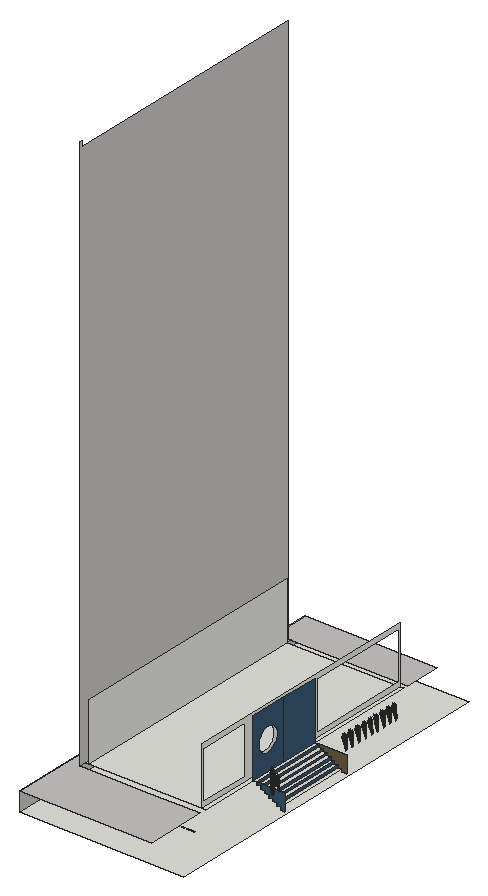
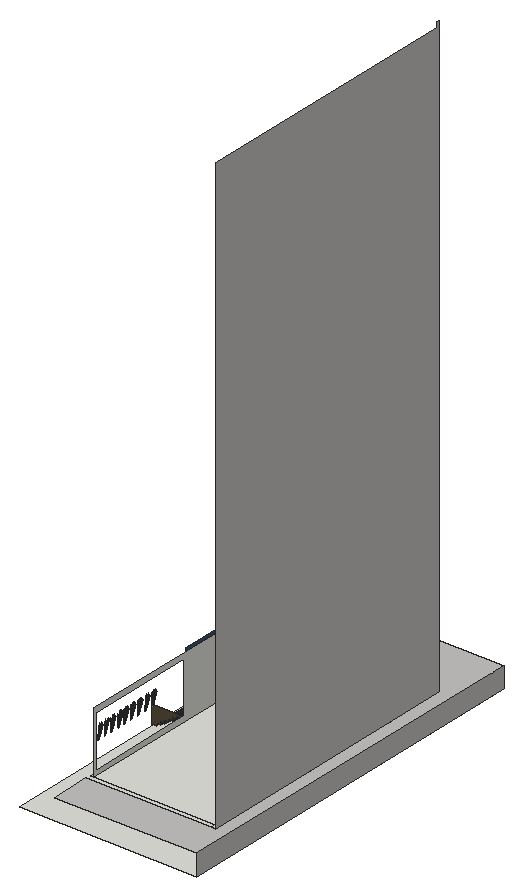
# SketchUp Ruby script. Lengths in inches.
U = 1.inch
M = Sketchup.active_model
def pt(a) = Geom::Point3d.new(a.map { |v| v * U })
def face(e, loops, mat)
  f = e.add_face(loops[0].map { |a| pt(a) })
  loops[1..].each { |l| e.add_face(l.map { |a| pt(a) }).erase! }
  f.material = f.back_material = mat if mat
  f
end
# faces: each face lists its corners as indices into pts; further lists are holes
def faces(e, pts, list, mat = nil) = list.each { |f| face(e, (f[0].is_a?(Array) ? f : [f]).map { |l| l.map { |i| pts[i] } }, mat) }
# xy, xz, yz: faces in a plane at the given z, y or x. An outline is a flat list of corners, or four numbers for a rectangle; further outlines are holes
def ring(l) = l.size == 4 ? [[l[0], l[1]], [l[2], l[1]], [l[2], l[3]], [l[0], l[3]]] : l.each_slice(2).to_a
def flat(e, list, mat, &to3) = list.each { |f| face(e, (f[0].is_a?(Array) ? f : [f]).map { |l| ring(l).map { |u, v| to3.(u, v) } }, mat) }
def xy(e, z, list, mat = nil) = flat(e, list, mat) { |x, y| [x, y, z] }
def xz(e, y, list, mat = nil) = flat(e, list, mat) { |x, z| [x, y, z] }
def yz(e, x, list, mat = nil) = flat(e, list, mat) { |y, z| [x, y, z] }
def lines(e, pts, list) = list.each { |a, b| e.add_line(pt(pts[a]), pt(pts[b])) }
# prism: a flat outline (further loops are holes) pulled along v
def prism(e, loops, v, mat = nil)
  f = face(e, loops, mat); d = Geom::Vector3d.new(v.map { |x| x * U })
  f.pushpull(f.normal.samedirection?(d) ? d.length : -d.length)
end
def box(e, o, s, mat = nil) = prism(e, [[o, [o[0] + s[0], o[1], o[2]], [o[0] + s[0], o[1] + s[1], o[2]], [o[0], o[1] + s[1], o[2]]]], [0, 0, s[2]], mat)
def at(x, y, z, deg = 0) = Geom::Transformation.translation(pt([x, y, z])) * Geom::Transformation.rotation(ORIGIN, Z_AXIS, deg.degrees)
def axes(o, x, y, z) = Geom::Transformation.new([*x, 0, *y, 0, *z, 0, *pt(o).to_a, 1])
def part(name) = M.definitions.add(name)
# library, detail: a bought-in or finely detailed component or shape, given as its bounding box
def library(name, o, s) = part(name).tap { |d| box(d.entities, o, s) }
def detail(e, o, s) = box(e.add_group.entities, o, s)
def put(e, d, t, mat = nil) = e.add_instance(d, t).tap { |i| i.material = mat if mat }
def group(e, t, mat = nil) = e.add_group.tap { |g| g.transformation = t; g.material = mat if mat }.entities
root = M.entities
M.materials.add("Carpet_01_1K").color = [196, 195, 193]
M.materials.add("Carpet_04_1K").color = [56, 85, 112]
M.materials.add("Forest_Floor_01_1K").color = [106, 91, 72]
M.materials.add("LightPink_Translucent").color = [144, 107, 117]
M.materials["LightPink_Translucent"].alpha = 0.75
M.materials.add("Marble_01_1K").color = [230, 221, 211]
c1 = part("blade")
p = [[2.15,0.21,22],[0,0.17,0],[0.09,0.45,0],[2.18,0.31,22],[2.29,0.31,22],[0.38,0.45,0],
  [2.48,0.24,33],[2.49,0.24,33],[2.48,0.22,33]]
faces(c1.entities,p,[[0,1,2,3],[4,5,2,3],[6,3,4,7],[8,0,3,6]])
c2 = part("seeds")
p = [[0.3,-0.1,1.38],[-0.01,-0.03,1.59],[-0.01,-0.03,0.03],[0.14,-0.07,-0.07],[0.29,-0.03,3],[0.15,0.01,3.11]]
faces(c2.entities,p,[[0,1,2,3],[1,0,4,5]],"LightPink_Translucent")
c3 = part("blade with seeds")
put(c3.entities,c1,at(0,0,0))
put(c3.entities,c2,axes([2.4,0.25,30.99],[1.5799,-0.05474,1.17369],[-0.12525,1.92788,0.29478],[-0.07173,-0.02425,1.56792]))
xy(root,-48,[[[0,0,410.57,890.67],[186.57,149.5,330.57,149.5,330.57,150.21,326.6875,151.48,317.8,153.17,308.78,153.74]]])
xy(root,-36,[[388.57,316.3,398.57,509.26]],"Marble_01_1K")
xy(root,-30,[[378.57,316.3,388.57,509.26]],"Marble_01_1K")
xy(root,-24,[[370.57,316.3,378.57,509.26]],"Marble_01_1K")
xy(root,-18,[[360.57,316.3,370.57,509.26]],"Marble_01_1K")
xy(root,-12,[[350.57,316.3,360.57,509.26]],"Marble_01_1K")
xy(root,-6,[[340.57,316.3,350.57,509.26]],"Marble_01_1K")
xy(root,0,[[30.57,167.5625,39.57,798.7],[39.57,167.5625,321.57,786.64],[321.57,167.5625,330.57,786.64]])
xy(root,0,[[0,0,330.57,0,330.57,149.5,186.57,149.5,186.57,149.51,30.57,149.51,30.57,798.7,330.57,798.7,330.57,890.67,0,890.67]],"Carpet_01_1K")
xy(root,0,[[330.57,316.3,340.57,509.26]],"Marble_01_1K")
xz(root,316.3,[[398.57,-42,398.57,-36,388.57,-36,388.57,-30,378.57,-30,378.57,-24,370.57,-24,370.57,-18,360.57,-18,360.57,-12,350.57,-12,350.57,-6,340.57,-6,340.57,0,410.57,0,410.57,-42]],"Carpet_04_1K")
xz(root,509.26,[[398.57,-42,410.57,-42,410.57,0,340.57,0,340.57,-6,350.57,-6,350.57,-12,360.57,-12,360.57,-18,370.57,-18,370.57,-24,378.57,-24,378.57,-30,388.57,-30,388.57,-36,398.57,-36]],"Forest_Floor_01_1K")
yz(root,0,[[0,-48,890.67,0]],"Carpet_01_1K")
yz(root,30.57,[[149.51,0,149.51,1398,155.5,1398,155.5,1386,798.7,1386,798.7,0]],"Carpet_01_1K")
yz(root,39.57,[[167.5625,0,786.64,144]])
yz(root,321.57,[[[167.5625,0,786.64,144],[525.34,12,782.62,132],[171.58,12,300.22,132],[361.46,41.77,365.23,41.79,368.97,42.28,372.61,43.24,376.11,44.64,379.4,46.47,382.43,48.7,385.17,51.3,387.55,54.21,389.55,57.41,391.14,60.82,392.29,64.41,392.97,68.12,393.1875,71.88,392.93,75.64,392.21,79.33,391.02,82.91,389.4,86.31,387.36,89.48,384.95,92.37,382.1875,94.93,379.13,97.13,375.82,98.93,372.31,100.3,368.65,101.22,364.91,101.67,361.15,101.65,357.41,101.16,353.77,100.2,350.27,98.79,346.98,96.96,343.94,94.73,341.21,92.14,338.82,89.22,336.82,86.03,335.24,82.61,334.09,79.02,333.41,75.32,333.1875,71.56,333.45,67.8,334.17,64.1,335.35,60.53,336.98,57.125,339.01,53.95,341.43,51.06,344.19,48.5,347.25,46.3,350.5625,44.5,354.07,43.14,357.72,42.22]]])
yz(root,330.57,[[[316.3,0,412.78,144],[361.46,41.77,357.72,42.22,354.07,43.14,350.5625,44.5,347.25,46.3,344.19,48.5,341.43,51.06,339.01,53.95,336.98,57.125,335.35,60.53,334.17,64.1,333.45,67.8,333.1875,71.56,333.41,75.32,334.09,79.02,335.24,82.61,336.82,86.03,338.82,89.22,341.21,92.14,343.94,94.73,346.98,96.96,350.27,98.79,353.77,100.2,357.41,101.16,361.15,101.65,364.91,101.67,368.65,101.22,372.31,100.3,375.82,98.93,379.13,97.13,382.1875,94.93,384.95,92.37,387.36,89.48,389.4,86.31,391.02,82.91,392.21,79.33,392.93,75.64,393.1875,71.88,392.97,68.12,392.29,64.41,391.14,60.82,389.55,57.41,387.55,54.21,385.17,51.3,382.43,48.7,379.4,46.47,376.11,44.64,372.61,43.24,368.97,42.28,365.23,41.79]],[412.78,0,509.26,144]],"Carpet_04_1K")
yz(root,340.57,[[316.3,-6,509.26,0]],"Carpet_04_1K")
yz(root,350.57,[[316.3,-12,509.26,-6]],"Carpet_04_1K")
yz(root,360.57,[[316.3,-18,509.26,-12]],"Carpet_04_1K")
yz(root,370.57,[[316.3,-24,509.26,-18]],"Carpet_04_1K")
yz(root,378.57,[[316.3,-30,509.26,-24]],"Carpet_04_1K")
yz(root,388.57,[[316.3,-36,509.26,-30]],"Carpet_04_1K")
put(root,c3,axes([397.55,292.79,3.875],[0.12246,-0.09864,1.71376],[0.1031,0.45582,0.13857],[-0.19225,0.10302,0.73262]))
put(root,c3,axes([397.17,293.5625,2.59],[0.12266,0.03828,1.43002],[0.07906,0.39104,-0.30754],[-0.16661,0.0732,0.61141]))
put(root,c3,axes([398.25,292.31,3.34],[0.10032,-0.06746,1.77064],[0.0346,0.47103,0.13857],[-0.2173,0.0625,0.63284]))
put(root,c3,axes([397.36,292.375,4.53],[-0.29332,-0.1301,-0.35414],[0.08555,-0.37955,0.4572],[-0.11809,0.0348,0.87481]))
put(root,c3,axes([397.56,292.57,4.68],[-0.09562,0.42421,-0.51099],[-0.32782,-0.1454,-0.3958],[-0.13199,0.0389,0.97773]))
put(root,c3,axes([397.4,292.54,1.49],[0.00895,0.0735,1.76342],[-0.18044,0.38382,-0.26939],[-0.12817,-0.01935,0.30037]))
put(root,c3,axes([396.91,294.38,2.77],[0.14709,-0.21136,1.1486],[0.05804,0.3346,0.84392],[-0.1063,0.05991,0.25299]))
put(root,c3,axes([398,293.09,3.875],[0.08815,-0.14329,1.71376],[0.22258,0.38678,0.13857],[-0.15267,0.17614,0.73262]))
put(root,c3,axes([397.47,293.47,4.53],[-0.30722,0.06665,-0.35414],[-0.08112,-0.381,0.4572],[-0.08804,0.10234,0.87481]))
put(root,c3,axes([397.3,294.6,1.49],[0.04734,0.04659,1.76342],[0.08027,0.4317,-0.26939],[-0.10492,0.09206,0.30037]))
put(root,c3,axes([397.93,293.45,3.875],[0.06572,-0.16029,1.71376],[0.27569,0.33172,0.13857],[-0.12437,0.20675,0.73262]))
put(root,c3,axes([397.72,293.51,4.68],[0.09067,0.42583,-0.51099],[-0.34336,0.07449,-0.3958],[-0.0984,0.11438,0.97773]))
put(root,c3,axes([398.58,293.21,2.06],[-0.36714,-0.07646,-0.62353],[0.07747,-0.47163,-0.16365],[-0.10956,-0.05715,1.37633]))
put(root,c3,axes([398.09,294.1,2.02],[-0.33032,-0.23318,-0.49651],[0.19744,-0.41812,0],[-0.07523,-0.05311,1.57504]))
put(root,c3,axes([398.3,294.38,2.375],[-0.22066,0.46731,0],[-0.36918,-0.26061,-0.51607],[-0.08408,-0.05936,1.63711]))
put(root,c3,axes([397.89,295.06,2.59],[0.11138,-0.07357,1.43002],[0.27499,0.22183,-0.30754],[-0.08185,0.19194,0.61141]))
put(root,c3,axes([398.99,293.28,2.67],[-0.35635,0.30962,-0.29095],[-0.23697,-0.43749,-0.50002],[-0.08792,-0.04443,1.59708]))
put(root,c3,axes([400.46,308.54,3.875],[0.14639,-0.01056,1.71376],[-0.09712,0.45778,0.13857],[-0.20862,-0.02831,0.73262]))
put(root,c3,axes([400.46,518.98,3.875],[0.14639,-0.01056,1.71376],[-0.09712,0.45778,0.13857],[-0.20862,-0.02831,0.73262]))
put(root,c3,axes([400.46,538.21,3.875],[0.14639,-0.01056,1.71376],[-0.09712,0.45778,0.13857],[-0.20862,-0.02831,0.73262]))
put(root,c3,axes([400.46,560.05,3.875],[0.14639,-0.01056,1.71376],[-0.09712,0.45778,0.13857],[-0.20862,-0.02831,0.73262]))
put(root,c3,axes([400.46,580.32,3.875],[0.14639,-0.01056,1.71376],[-0.09712,0.45778,0.13857],[-0.20862,-0.02831,0.73262]))
put(root,c3,axes([400.46,599.76,3.875],[0.14639,-0.01056,1.71376],[-0.09712,0.45778,0.13857],[-0.20862,-0.02831,0.73262]))
put(root,c3,axes([400.46,617.34,3.875],[0.14639,-0.01056,1.71376],[-0.09712,0.45778,0.13857],[-0.20862,-0.02831,0.73262]))
put(root,c3,axes([400.46,637.875,3.875],[0.14639,-0.01056,1.71376],[-0.09712,0.45778,0.13857],[-0.20862,-0.02831,0.73262]))
put(root,c3,axes([400.46,656.55,3.875],[0.14639,-0.01056,1.71376],[-0.09712,0.45778,0.13857],[-0.20862,-0.02831,0.73262]))
put(root,c3,axes([400.46,674.76,3.875],[0.14639,-0.01056,1.71376],[-0.09712,0.45778,0.13857],[-0.20862,-0.02831,0.73262]))
put(root,c3,axes([398.1875,293.93,2.03],[-0.08291,-0.40636,-0.30978],[0.32928,-0.11539,0.30978],[-0.06638,-0.04686,1.38974]))
put(root,c3,axes([398.01,294.35,4.53],[-0.23881,0.24554,-0.35414],[-0.22606,-0.28036,0.4572],[-0.0344,0.14245,0.87481]))
put(root,c3,axes([399.23,293.61,2.06],[-0.23773,0.35053,-0.62353],[-0.29532,-0.31785,-0.16365],[-0.09526,0.08744,1.37633]))
put(root,c3,axes([400.52,309.35,3.875],[0.12246,-0.09864,1.71376],[0.1031,0.45582,0.13857],[-0.19225,0.10302,0.73262]))
put(root,c3,axes([400.52,519.79,3.875],[0.12246,-0.09864,1.71376],[0.1031,0.45582,0.13857],[-0.19225,0.10302,0.73262]))
put(root,c3,axes([400.52,539.01,3.875],[0.12246,-0.09864,1.71376],[0.1031,0.45582,0.13857],[-0.19225,0.10302,0.73262]))
put(root,c3,axes([400.52,560.86,3.875],[0.12246,-0.09864,1.71376],[0.1031,0.45582,0.13857],[-0.19225,0.10302,0.73262]))
put(root,c3,axes([400.52,581.125,3.875],[0.12246,-0.09864,1.71376],[0.1031,0.45582,0.13857],[-0.19225,0.10302,0.73262]))
put(root,c3,axes([400.52,600.5625,3.875],[0.12246,-0.09864,1.71376],[0.1031,0.45582,0.13857],[-0.19225,0.10302,0.73262]))
put(root,c3,axes([400.52,618.15,3.875],[0.12246,-0.09864,1.71376],[0.1031,0.45582,0.13857],[-0.19225,0.10302,0.73262]))
put(root,c3,axes([400.52,638.68,3.875],[0.12246,-0.09864,1.71376],[0.1031,0.45582,0.13857],[-0.19225,0.10302,0.73262]))
put(root,c3,axes([400.52,657.35,3.875],[0.12246,-0.09864,1.71376],[0.1031,0.45582,0.13857],[-0.19225,0.10302,0.73262]))
put(root,c3,axes([400.52,675.57,3.875],[0.12246,-0.09864,1.71376],[0.1031,0.45582,0.13857],[-0.19225,0.10302,0.73262]))
put(root,c3,axes([399.39,293.42,2.46],[-0.34464,-0.37536,-0.25192],[0.29,-0.42149,0.5513],[-0.0928,0.04391,1.68216]))
put(root,c3,axes([398.77,293.06,2.21],[-0.21202,-0.39143,-0.44739],[0.32115,-0.27564,0.21531],[-0.06861,-0.04843,1.43643]))
put(root,c3,axes([400.14,310.125,2.59],[0.12266,0.03828,1.43002],[0.07906,0.39104,-0.30754],[-0.16661,0.0732,0.61141]))
put(root,c3,axes([400.14,520.5625,2.59],[0.12266,0.03828,1.43002],[0.07906,0.39104,-0.30754],[-0.16661,0.0732,0.61141]))
put(root,c3,axes([400.14,539.79,2.59],[0.12266,0.03828,1.43002],[0.07906,0.39104,-0.30754],[-0.16661,0.0732,0.61141]))
put(root,c3,axes([400.14,561.64,2.59],[0.12266,0.03828,1.43002],[0.07906,0.39104,-0.30754],[-0.16661,0.0732,0.61141]))
put(root,c3,axes([400.14,581.9,2.59],[0.12266,0.03828,1.43002],[0.07906,0.39104,-0.30754],[-0.16661,0.0732,0.61141]))
put(root,c3,axes([400.14,601.34,2.59],[0.12266,0.03828,1.43002],[0.07906,0.39104,-0.30754],[-0.16661,0.0732,0.61141]))
put(root,c3,axes([400.14,618.92,2.59],[0.12266,0.03828,1.43002],[0.07906,0.39104,-0.30754],[-0.16661,0.0732,0.61141]))
put(root,c3,axes([400.14,639.46,2.59],[0.12266,0.03828,1.43002],[0.07906,0.39104,-0.30754],[-0.16661,0.0732,0.61141]))
put(root,c3,axes([400.14,658.13,2.59],[0.12266,0.03828,1.43002],[0.07906,0.39104,-0.30754],[-0.16661,0.0732,0.61141]))
put(root,c3,axes([400.14,676.35,2.59],[0.12266,0.03828,1.43002],[0.07906,0.39104,-0.30754],[-0.16661,0.0732,0.61141]))
put(root,c3,axes([398.17,294.09,5.34],[-0.00918,0.43138,-0.7886],[-0.38672,-0.02897,0.09517],[-0.04081,0.18275,1.11556]))
put(root,c3,axes([398.16,295.3,2.77],[-0.00913,-0.2773,1.1486],[0.22824,0.19778,0.84392],[-0.04489,0.13217,0.25299]))
put(root,c3,axes([399.22,293.34,2.21],[-0.38326,0.02879,-0.44739],[-0.03466,-0.47788,0.21531],[-0.06861,0.04843,1.43643]))
put(root,c3,axes([401.22,308.875,3.34],[0.10032,-0.06746,1.77064],[0.0346,0.47103,0.13857],[-0.2173,0.0625,0.63284]))
put(root,c3,axes([401.22,519.31,3.34],[0.10032,-0.06746,1.77064],[0.0346,0.47103,0.13857],[-0.2173,0.0625,0.63284]))
put(root,c3,axes([401.22,538.54,3.34],[0.10032,-0.06746,1.77064],[0.0346,0.47103,0.13857],[-0.2173,0.0625,0.63284]))
put(root,c3,axes([401.22,560.38,3.34],[0.10032,-0.06746,1.77064],[0.0346,0.47103,0.13857],[-0.2173,0.0625,0.63284]))
put(root,c3,axes([401.22,580.65,3.34],[0.10032,-0.06746,1.77064],[0.0346,0.47103,0.13857],[-0.2173,0.0625,0.63284]))
put(root,c3,axes([401.22,600.09,3.34],[0.10032,-0.06746,1.77064],[0.0346,0.47103,0.13857],[-0.2173,0.0625,0.63284]))
put(root,c3,axes([401.22,617.67,3.34],[0.10032,-0.06746,1.77064],[0.0346,0.47103,0.13857],[-0.2173,0.0625,0.63284]))
put(root,c3,axes([401.22,638.21,3.34],[0.10032,-0.06746,1.77064],[0.0346,0.47103,0.13857],[-0.2173,0.0625,0.63284]))
put(root,c3,axes([401.22,656.88,3.34],[0.10032,-0.06746,1.77064],[0.0346,0.47103,0.13857],[-0.2173,0.0625,0.63284]))
put(root,c3,axes([401.22,675.09,3.34],[0.10032,-0.06746,1.77064],[0.0346,0.47103,0.13857],[-0.2173,0.0625,0.63284]))
put(root,c3,axes([398.49,294.14,2.48],[0.33032,0.23318,0.49651],[-0.19744,0.41812,0],[-0.07523,-0.05311,1.57504]))
put(root,c3,axes([398.04,294.7,3.36],[0.00775,-0.24075,1.54345],[0.34877,0.12716,0.21329],[-0.03022,0.25658,0.72882]))
put(root,c3,axes([400.89,308.12,4.98],[-0.35281,-0.01123,-0.71045],[0.0237,-0.47284,0.08574],[-0.14947,-0.0499,1.00501]))
put(root,c3,axes([400.89,518.55,4.98],[-0.35281,-0.01123,-0.71045],[0.0237,-0.47284,0.08574],[-0.14947,-0.0499,1.00501]))
put(root,c3,axes([400.89,537.78,4.98],[-0.35281,-0.01123,-0.71045],[0.0237,-0.47284,0.08574],[-0.14947,-0.0499,1.00501]))
put(root,c3,axes([400.89,559.63,4.98],[-0.35281,-0.01123,-0.71045],[0.0237,-0.47284,0.08574],[-0.14947,-0.0499,1.00501]))
put(root,c3,axes([400.89,579.9,4.98],[-0.35281,-0.01123,-0.71045],[0.0237,-0.47284,0.08574],[-0.14947,-0.0499,1.00501]))
put(root,c3,axes([400.89,599.33,4.98],[-0.35281,-0.01123,-0.71045],[0.0237,-0.47284,0.08574],[-0.14947,-0.0499,1.00501]))
put(root,c3,axes([400.89,616.92,4.98],[-0.35281,-0.01123,-0.71045],[0.0237,-0.47284,0.08574],[-0.14947,-0.0499,1.00501]))
put(root,c3,axes([400.89,637.45,4.98],[-0.35281,-0.01123,-0.71045],[0.0237,-0.47284,0.08574],[-0.14947,-0.0499,1.00501]))
put(root,c3,axes([400.89,656.125,4.98],[-0.35281,-0.01123,-0.71045],[0.0237,-0.47284,0.08574],[-0.14947,-0.0499,1.00501]))
put(root,c3,axes([400.89,674.34,4.98],[-0.35281,-0.01123,-0.71045],[0.0237,-0.47284,0.08574],[-0.14947,-0.0499,1.00501]))
put(root,c3,axes([398.96,293.41,2.62],[-0.06809,0.4162,0.1448],[-0.33266,-0.07225,-0.41347],[-0.06054,-0.04274,1.26744]))
put(root,c3,axes([400.61,308.23,2.59],[0.06891,0.12984,1.43002],[-0.15879,0.35293,-0.30754],[-0.16304,-0.08436,0.61141]))
put(root,c3,axes([400.61,518.67,2.59],[0.06891,0.12984,1.43002],[-0.15879,0.35293,-0.30754],[-0.16304,-0.08436,0.61141]))
put(root,c3,axes([400.61,537.9,2.59],[0.06891,0.12984,1.43002],[-0.15879,0.35293,-0.30754],[-0.16304,-0.08436,0.61141]))
put(root,c3,axes([400.61,559.74,2.59],[0.06891,0.12984,1.43002],[-0.15879,0.35293,-0.30754],[-0.16304,-0.08436,0.61141]))
put(root,c3,axes([400.61,580.01,2.59],[0.06891,0.12984,1.43002],[-0.15879,0.35293,-0.30754],[-0.16304,-0.08436,0.61141]))
put(root,c3,axes([400.61,599.45,2.59],[0.06891,0.12984,1.43002],[-0.15879,0.35293,-0.30754],[-0.16304,-0.08436,0.61141]))
put(root,c3,axes([400.61,617.03,2.59],[0.06891,0.12984,1.43002],[-0.15879,0.35293,-0.30754],[-0.16304,-0.08436,0.61141]))
put(root,c3,axes([400.61,637.56,2.59],[0.06891,0.12984,1.43002],[-0.15879,0.35293,-0.30754],[-0.16304,-0.08436,0.61141]))
put(root,c3,axes([400.61,656.24,2.59],[0.06891,0.12984,1.43002],[-0.15879,0.35293,-0.30754],[-0.16304,-0.08436,0.61141]))
put(root,c3,axes([400.61,674.45,2.59],[0.06891,0.12984,1.43002],[-0.15879,0.35293,-0.30754],[-0.16304,-0.08436,0.61141]))
put(root,c3,axes([399.62,294.57,2.02],[-0.33032,0.23318,-0.49651],[-0.19744,-0.41812,0],[-0.07523,0.05311,1.57504]))
put(root,c3,axes([399.64,294.45,2.19],[-0.21791,-0.46895,-0.05142],[0.36918,-0.26061,0.51607],[-0.09097,0.04465,1.6363]))
put(root,c3,axes([400.33,308.9375,4.53],[-0.29332,-0.1301,-0.35414],[0.08555,-0.37955,0.4572],[-0.11809,0.0348,0.87481]))
put(root,c3,axes([400.33,519.375,4.53],[-0.29332,-0.1301,-0.35414],[0.08555,-0.37955,0.4572],[-0.11809,0.0348,0.87481]))
put(root,c3,axes([400.33,538.6,4.53],[-0.29332,-0.1301,-0.35414],[0.08555,-0.37955,0.4572],[-0.11809,0.0348,0.87481]))
put(root,c3,axes([400.33,560.45,4.53],[-0.29332,-0.1301,-0.35414],[0.08555,-0.37955,0.4572],[-0.11809,0.0348,0.87481]))
put(root,c3,axes([400.33,580.71,4.53],[-0.29332,-0.1301,-0.35414],[0.08555,-0.37955,0.4572],[-0.11809,0.0348,0.87481]))
put(root,c3,axes([400.33,600.15,4.53],[-0.29332,-0.1301,-0.35414],[0.08555,-0.37955,0.4572],[-0.11809,0.0348,0.87481]))
put(root,c3,axes([400.33,617.73,4.53],[-0.29332,-0.1301,-0.35414],[0.08555,-0.37955,0.4572],[-0.11809,0.0348,0.87481]))
put(root,c3,axes([400.33,638.27,4.53],[-0.29332,-0.1301,-0.35414],[0.08555,-0.37955,0.4572],[-0.11809,0.0348,0.87481]))
put(root,c3,axes([400.33,656.94,4.53],[-0.29332,-0.1301,-0.35414],[0.08555,-0.37955,0.4572],[-0.11809,0.0348,0.87481]))
put(root,c3,axes([400.33,675.16,4.53],[-0.29332,-0.1301,-0.35414],[0.08555,-0.37955,0.4572],[-0.11809,0.0348,0.87481]))
put(root,c3,axes([400.73,307.81,3.875],[0.1311,0.08035,1.71376],[-0.27131,0.33708,0.13857],[-0.16909,-0.15206,0.73262]))
put(root,c3,axes([400.73,518.25,3.875],[0.1311,0.08035,1.71376],[-0.27131,0.33708,0.13857],[-0.16909,-0.15206,0.73262]))
put(root,c3,axes([400.73,537.47,3.875],[0.1311,0.08035,1.71376],[-0.27131,0.33708,0.13857],[-0.16909,-0.15206,0.73262]))
put(root,c3,axes([400.73,559.32,3.875],[0.1311,0.08035,1.71376],[-0.27131,0.33708,0.13857],[-0.16909,-0.15206,0.73262]))
put(root,c3,axes([400.73,579.59,3.875],[0.1311,0.08035,1.71376],[-0.27131,0.33708,0.13857],[-0.16909,-0.15206,0.73262]))
put(root,c3,axes([400.73,599.02,3.875],[0.1311,0.08035,1.71376],[-0.27131,0.33708,0.13857],[-0.16909,-0.15206,0.73262]))
put(root,c3,axes([400.73,616.61,3.875],[0.1311,0.08035,1.71376],[-0.27131,0.33708,0.13857],[-0.16909,-0.15206,0.73262]))
put(root,c3,axes([400.73,637.14,3.875],[0.1311,0.08035,1.71376],[-0.27131,0.33708,0.13857],[-0.16909,-0.15206,0.73262]))
put(root,c3,axes([400.73,655.8125,3.875],[0.1311,0.08035,1.71376],[-0.27131,0.33708,0.13857],[-0.16909,-0.15206,0.73262]))
put(root,c3,axes([400.73,674.03,3.875],[0.1311,0.08035,1.71376],[-0.27131,0.33708,0.13857],[-0.16909,-0.15206,0.73262]))
put(root,c3,axes([398.24,294.23,5],[0.25266,0.31335,-0.5672],[-0.2669,0.27442,-0.43934],[-0.03844,0.15921,1.08528]))
put(root,c3,axes([399.54,294.39,2.03],[-0.32928,-0.11539,-0.30978],[0.08291,-0.40636,0.30978],[-0.06638,0.04686,1.38974]))
put(root,c3,axes([400.53,309.13,4.68],[-0.09562,0.42421,-0.51099],[-0.32782,-0.1454,-0.3958],[-0.13199,0.0389,0.97773]))
put(root,c3,axes([400.53,519.57,4.68],[-0.09562,0.42421,-0.51099],[-0.32782,-0.1454,-0.3958],[-0.13199,0.0389,0.97773]))
put(root,c3,axes([400.53,538.79,4.68],[-0.09562,0.42421,-0.51099],[-0.32782,-0.1454,-0.3958],[-0.13199,0.0389,0.97773]))
put(root,c3,axes([400.53,560.64,4.68],[-0.09562,0.42421,-0.51099],[-0.32782,-0.1454,-0.3958],[-0.13199,0.0389,0.97773]))
put(root,c3,axes([400.53,580.91,4.68],[-0.09562,0.42421,-0.51099],[-0.32782,-0.1454,-0.3958],[-0.13199,0.0389,0.97773]))
put(root,c3,axes([400.53,600.34,4.68],[-0.09562,0.42421,-0.51099],[-0.32782,-0.1454,-0.3958],[-0.13199,0.0389,0.97773]))
put(root,c3,axes([400.53,617.93,4.68],[-0.09562,0.42421,-0.51099],[-0.32782,-0.1454,-0.3958],[-0.13199,0.0389,0.97773]))
put(root,c3,axes([400.53,638.46,4.68],[-0.09562,0.42421,-0.51099],[-0.32782,-0.1454,-0.3958],[-0.13199,0.0389,0.97773]))
put(root,c3,axes([400.53,657.14,4.68],[-0.09562,0.42421,-0.51099],[-0.32782,-0.1454,-0.3958],[-0.13199,0.0389,0.97773]))
put(root,c3,axes([400.53,675.35,4.68],[-0.09562,0.42421,-0.51099],[-0.32782,-0.1454,-0.3958],[-0.13199,0.0389,0.97773]))
put(root,c3,axes([399.73,292.65,2.84],[-0.00964,-0.43909,1.41272],[0.43635,0.11382,0.59816],[-0.1032,0.24027,1.3335]))
put(root,c3,axes([400.78,308.21,4.68],[-0.25628,0.30892,-0.51099],[-0.22444,-0.32634,-0.3958],[-0.13021,-0.047,0.97773]))
put(root,c3,axes([400.78,518.65,4.68],[-0.25628,0.30892,-0.51099],[-0.22444,-0.32634,-0.3958],[-0.13021,-0.047,0.97773]))
put(root,c3,axes([400.78,537.88,4.68],[-0.25628,0.30892,-0.51099],[-0.22444,-0.32634,-0.3958],[-0.13021,-0.047,0.97773]))
put(root,c3,axes([400.78,559.72,4.68],[-0.25628,0.30892,-0.51099],[-0.22444,-0.32634,-0.3958],[-0.13021,-0.047,0.97773]))
put(root,c3,axes([400.78,579.99,4.68],[-0.25628,0.30892,-0.51099],[-0.22444,-0.32634,-0.3958],[-0.13021,-0.047,0.97773]))
put(root,c3,axes([400.78,599.43,4.68],[-0.25628,0.30892,-0.51099],[-0.22444,-0.32634,-0.3958],[-0.13021,-0.047,0.97773]))
put(root,c3,axes([400.78,617.01,4.68],[-0.25628,0.30892,-0.51099],[-0.22444,-0.32634,-0.3958],[-0.13021,-0.047,0.97773]))
put(root,c3,axes([400.78,637.55,4.68],[-0.25628,0.30892,-0.51099],[-0.22444,-0.32634,-0.3958],[-0.13021,-0.047,0.97773]))
put(root,c3,axes([400.78,656.22,4.68],[-0.25628,0.30892,-0.51099],[-0.22444,-0.32634,-0.3958],[-0.13021,-0.047,0.97773]))
put(root,c3,axes([400.78,674.43,4.68],[-0.25628,0.30892,-0.51099],[-0.22444,-0.32634,-0.3958],[-0.13021,-0.047,0.97773]))
put(root,c3,axes([400.36,309.1,1.49],[0.00895,0.0735,1.76342],[-0.18044,0.38382,-0.26939],[-0.12817,-0.01935,0.30037]))
put(root,c3,axes([400.36,519.54,1.49],[0.00895,0.0735,1.76342],[-0.18044,0.38382,-0.26939],[-0.12817,-0.01935,0.30037]))
put(root,c3,axes([400.36,538.77,1.49],[0.00895,0.0735,1.76342],[-0.18044,0.38382,-0.26939],[-0.12817,-0.01935,0.30037]))
put(root,c3,axes([400.36,560.61,1.49],[0.00895,0.0735,1.76342],[-0.18044,0.38382,-0.26939],[-0.12817,-0.01935,0.30037]))
put(root,c3,axes([400.36,580.88,1.49],[0.00895,0.0735,1.76342],[-0.18044,0.38382,-0.26939],[-0.12817,-0.01935,0.30037]))
put(root,c3,axes([400.36,600.32,1.49],[0.00895,0.0735,1.76342],[-0.18044,0.38382,-0.26939],[-0.12817,-0.01935,0.30037]))
put(root,c3,axes([400.36,617.9,1.49],[0.00895,0.0735,1.76342],[-0.18044,0.38382,-0.26939],[-0.12817,-0.01935,0.30037]))
put(root,c3,axes([400.36,638.4375,1.49],[0.00895,0.0735,1.76342],[-0.18044,0.38382,-0.26939],[-0.12817,-0.01935,0.30037]))
put(root,c3,axes([400.36,657.11,1.49],[0.00895,0.0735,1.76342],[-0.18044,0.38382,-0.26939],[-0.12817,-0.01935,0.30037]))
put(root,c3,axes([400.36,675.32,1.49],[0.00895,0.0735,1.76342],[-0.18044,0.38382,-0.26939],[-0.12817,-0.01935,0.30037]))
put(root,c3,axes([397.97,294.7,2.82],[0.32063,-0.08258,0.06507],[0.07371,0.33271,-0.86304],[-0.02033,0.16842,0.7736]))
put(root,c3,axes([399.49,293.21,2.67],[0.04113,0.53214,-0.29095],[-0.42835,0.03218,-0.50002],[-0.07543,0.07088,1.59708]))
put(root,c3,axes([398.53,293.78,3.875],[-0.00864,-0.17899,1.71376],[0.37441,0.11874,0.13857],[-0.02316,0.25508,0.73262]))
put(root,c3,axes([399.88,310.95,2.77],[0.14709,-0.21136,1.1486],[0.05804,0.3346,0.84392],[-0.1063,0.05991,0.25299]))
put(root,c3,axes([399.88,521.38,2.77],[0.14709,-0.21136,1.1486],[0.05804,0.3346,0.84392],[-0.1063,0.05991,0.25299]))
put(root,c3,axes([399.88,540.61,2.77],[0.14709,-0.21136,1.1486],[0.05804,0.3346,0.84392],[-0.1063,0.05991,0.25299]))
put(root,c3,axes([399.88,562.45,2.77],[0.14709,-0.21136,1.1486],[0.05804,0.3346,0.84392],[-0.1063,0.05991,0.25299]))
put(root,c3,axes([399.88,582.72,2.77],[0.14709,-0.21136,1.1486],[0.05804,0.3346,0.84392],[-0.1063,0.05991,0.25299]))
put(root,c3,axes([399.88,602.16,2.77],[0.14709,-0.21136,1.1486],[0.05804,0.3346,0.84392],[-0.1063,0.05991,0.25299]))
put(root,c3,axes([399.88,619.74,2.77],[0.14709,-0.21136,1.1486],[0.05804,0.3346,0.84392],[-0.1063,0.05991,0.25299]))
put(root,c3,axes([399.88,640.28,2.77],[0.14709,-0.21136,1.1486],[0.05804,0.3346,0.84392],[-0.1063,0.05991,0.25299]))
put(root,c3,axes([399.88,658.95,2.77],[0.14709,-0.21136,1.1486],[0.05804,0.3346,0.84392],[-0.1063,0.05991,0.25299]))
put(root,c3,axes([399.88,677.17,2.77],[0.14709,-0.21136,1.1486],[0.05804,0.3346,0.84392],[-0.1063,0.05991,0.25299]))
put(root,c3,axes([398.85,293.02,2.36],[0.44609,0.09826,0.45755],[-0.09078,0.55493,0.17955],[-0.06519,-0.05359,1.58856]))
put(root,c3,axes([400.68,307.92,4.53],[-0.20082,-0.29199,-0.35414],[0.2293,-0.2764,0.4572],[-0.1165,-0.04206,0.87481]))
put(root,c3,axes([400.68,518.36,4.53],[-0.20082,-0.29199,-0.35414],[0.2293,-0.2764,0.4572],[-0.1165,-0.04206,0.87481]))
put(root,c3,axes([400.68,537.59,4.53],[-0.20082,-0.29199,-0.35414],[0.2293,-0.2764,0.4572],[-0.1165,-0.04206,0.87481]))
put(root,c3,axes([400.68,559.43,4.53],[-0.20082,-0.29199,-0.35414],[0.2293,-0.2764,0.4572],[-0.1165,-0.04206,0.87481]))
put(root,c3,axes([400.68,579.7,4.53],[-0.20082,-0.29199,-0.35414],[0.2293,-0.2764,0.4572],[-0.1165,-0.04206,0.87481]))
put(root,c3,axes([400.68,599.14,4.53],[-0.20082,-0.29199,-0.35414],[0.2293,-0.2764,0.4572],[-0.1165,-0.04206,0.87481]))
put(root,c3,axes([400.68,616.72,4.53],[-0.20082,-0.29199,-0.35414],[0.2293,-0.2764,0.4572],[-0.1165,-0.04206,0.87481]))
put(root,c3,axes([400.68,637.26,4.53],[-0.20082,-0.29199,-0.35414],[0.2293,-0.2764,0.4572],[-0.1165,-0.04206,0.87481]))
put(root,c3,axes([400.68,655.93,4.53],[-0.20082,-0.29199,-0.35414],[0.2293,-0.2764,0.4572],[-0.1165,-0.04206,0.87481]))
put(root,c3,axes([400.68,674.14,4.53],[-0.20082,-0.29199,-0.35414],[0.2293,-0.2764,0.4572],[-0.1165,-0.04206,0.87481]))
put(root,c3,axes([400.97,309.66,3.875],[0.08815,-0.14329,1.71376],[0.22258,0.38678,0.13857],[-0.15267,0.17614,0.73262]))
put(root,c3,axes([400.97,520.09,3.875],[0.08815,-0.14329,1.71376],[0.22258,0.38678,0.13857],[-0.15267,0.17614,0.73262]))
put(root,c3,axes([400.97,539.32,3.875],[0.08815,-0.14329,1.71376],[0.22258,0.38678,0.13857],[-0.15267,0.17614,0.73262]))
put(root,c3,axes([400.97,561.17,3.875],[0.08815,-0.14329,1.71376],[0.22258,0.38678,0.13857],[-0.15267,0.17614,0.73262]))
put(root,c3,axes([400.97,581.43,3.875],[0.08815,-0.14329,1.71376],[0.22258,0.38678,0.13857],[-0.15267,0.17614,0.73262]))
put(root,c3,axes([400.97,600.87,3.875],[0.08815,-0.14329,1.71376],[0.22258,0.38678,0.13857],[-0.15267,0.17614,0.73262]))
put(root,c3,axes([400.97,618.45,3.875],[0.08815,-0.14329,1.71376],[0.22258,0.38678,0.13857],[-0.15267,0.17614,0.73262]))
put(root,c3,axes([400.97,638.99,3.875],[0.08815,-0.14329,1.71376],[0.22258,0.38678,0.13857],[-0.15267,0.17614,0.73262]))
put(root,c3,axes([400.97,657.66,3.875],[0.08815,-0.14329,1.71376],[0.22258,0.38678,0.13857],[-0.15267,0.17614,0.73262]))
put(root,c3,axes([400.97,675.875,3.875],[0.08815,-0.14329,1.71376],[0.22258,0.38678,0.13857],[-0.15267,0.17614,0.73262]))
put(root,c3,axes([400.43,310.03,4.53],[-0.30722,0.06665,-0.35414],[-0.08112,-0.381,0.4572],[-0.08804,0.10234,0.87481]))
put(root,c3,axes([400.43,520.47,4.53],[-0.30722,0.06665,-0.35414],[-0.08112,-0.381,0.4572],[-0.08804,0.10234,0.87481]))
put(root,c3,axes([400.43,539.7,4.53],[-0.30722,0.06665,-0.35414],[-0.08112,-0.381,0.4572],[-0.08804,0.10234,0.87481]))
put(root,c3,axes([400.43,561.54,4.53],[-0.30722,0.06665,-0.35414],[-0.08112,-0.381,0.4572],[-0.08804,0.10234,0.87481]))
put(root,c3,axes([400.43,581.81,4.53],[-0.30722,0.06665,-0.35414],[-0.08112,-0.381,0.4572],[-0.08804,0.10234,0.87481]))
put(root,c3,axes([400.43,601.24,4.53],[-0.30722,0.06665,-0.35414],[-0.08112,-0.381,0.4572],[-0.08804,0.10234,0.87481]))
